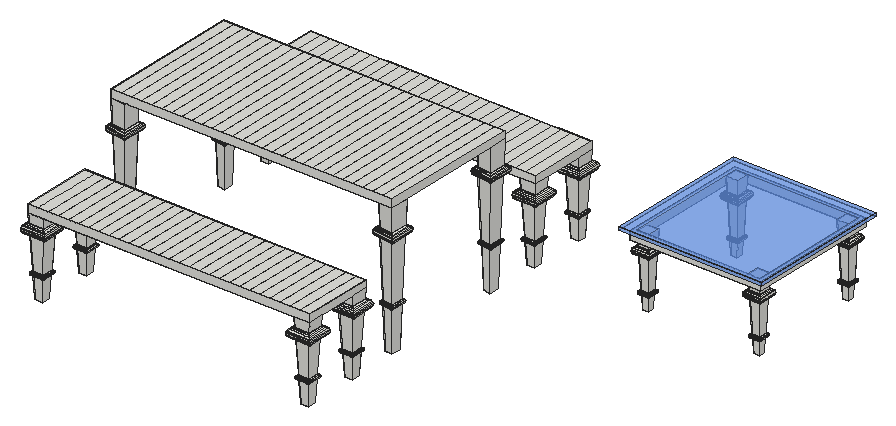
# SketchUp Ruby script. Lengths in millimetres.
U = 1.mm
M = Sketchup.active_model
def pt(a) = Geom::Point3d.new(a.map { |v| v * U })
def face(e, loops, mat)
  f = e.add_face(loops[0].map { |a| pt(a) })
  loops[1..].each { |l| e.add_face(l.map { |a| pt(a) }).erase! }
  f.material = f.back_material = mat if mat
  f
end
# faces: each face lists its corners as indices into pts; further lists are holes
def faces(e, pts, list, mat = nil) = list.each { |f| face(e, (f[0].is_a?(Array) ? f : [f]).map { |l| l.map { |i| pts[i] } }, mat) }
# xy, xz, yz: faces in a plane at the given z, y or x. An outline is a flat list of corners, or four numbers for a rectangle; further outlines are holes
def ring(l) = l.size == 4 ? [[l[0], l[1]], [l[2], l[1]], [l[2], l[3]], [l[0], l[3]]] : l.each_slice(2).to_a
def flat(e, list, mat, &to3) = list.each { |f| face(e, (f[0].is_a?(Array) ? f : [f]).map { |l| ring(l).map { |u, v| to3.(u, v) } }, mat) }
def xy(e, z, list, mat = nil) = flat(e, list, mat) { |x, y| [x, y, z] }
def xz(e, y, list, mat = nil) = flat(e, list, mat) { |x, z| [x, y, z] }
def yz(e, x, list, mat = nil) = flat(e, list, mat) { |y, z| [x, y, z] }
def lines(e, pts, list) = list.each { |a, b| e.add_line(pt(pts[a]), pt(pts[b])) }
# prism: a flat outline (further loops are holes) pulled along v
def prism(e, loops, v, mat = nil)
  f = face(e, loops, mat); d = Geom::Vector3d.new(v.map { |x| x * U })
  f.pushpull(f.normal.samedirection?(d) ? d.length : -d.length)
end
def box(e, o, s, mat = nil) = prism(e, [[o, [o[0] + s[0], o[1], o[2]], [o[0] + s[0], o[1] + s[1], o[2]], [o[0], o[1] + s[1], o[2]]]], [0, 0, s[2]], mat)
def at(x, y, z, deg = 0) = Geom::Transformation.translation(pt([x, y, z])) * Geom::Transformation.rotation(ORIGIN, Z_AXIS, deg.degrees)
def axes(o, x, y, z) = Geom::Transformation.new([*x, 0, *y, 0, *z, 0, *pt(o).to_a, 1])
def part(name) = M.definitions.add(name)
# library, detail: a bought-in or finely detailed component or shape, given as its bounding box
def library(name, o, s) = part(name).tap { |d| box(d.entities, o, s) }
def detail(e, o, s) = box(e.add_group.entities, o, s)
def put(e, d, t, mat = nil) = e.add_instance(d, t).tap { |i| i.material = mat if mat }
def group(e, t, mat = nil) = e.add_group.tap { |g| g.transformation = t; g.material = mat if mat }.entities
root = M.entities
M.materials.add("[Translucent Glass Blue]").color = [100, 149, 237]
M.materials["[Translucent Glass Blue]"].alpha = 0.5
c1 = part("Table leg \#1")
xy(c1.entities,0,[[95.2,52.8,45.9,59.8,45.9,113.1,95.7,113.1]])
xy(c1.entities,858,[[120,24.1,120.9,138.1,20.9,138.1,20.9,38.1]])
p = [[38.2,53.1,264.1],[45.9,59.8,0],[95.2,52.8,0],[102.8,44,264.1],[95.7,113.1,0],[103.5,120.8,264.1],
  [38.2,120.8,264.1],[45.9,113.1,0],[34.7,50,264.4],[37.9,52.8,264],[103.2,43.6,264],[106.4,39.8,264.4],
  [103.9,121.1,264],[107.1,124.4,264.4],[34.7,124.4,264.4],[37.9,121.1,264],[31.6,47.3,265.7],[109.4,36.4,265.7],
  [110.2,127.4,265.7],[31.6,127.4,265.7],[29,45.1,267.7],[111.9,33.4,267.7],[112.8,130,267.7],[29,130,267.7],
  [27.1,43.4,270.2],[113.9,31.1,270.2],[114.8,131.9,270.2],[27.1,131.9,270.2],[25.8,42.3,273.3],[115.1,29.7,273.3],
  [116,133.2,273.3],[25.8,133.2,273.3],[25.4,41.9,276.5],[115.6,29.2,276.5],[116.5,133.6,276.5],[25.4,133.6,276.5],
  [25.8,42.3,279.7],[115.1,29.7,279.7],[116,133.2,279.7],[25.8,133.2,279.7],[27.1,43.4,282.7],[113.9,31.1,282.7],
  [114.8,131.9,282.7],[27.1,131.9,282.7],[29,45.1,285.3],[111.9,33.4,285.3],[112.8,130,285.3],[29,130,285.3],
  [31.6,47.3,287.3],[109.4,36.4,287.3],[110.2,127.4,287.3],[31.6,127.4,287.3],[34.7,50,288.6],[106.4,39.8,288.6],
  [107.1,124.4,288.6],[34.7,124.4,288.6],[37.5,52.5,288.9],[103.5,43.1,288.9],[104.2,121.5,288.9],[37.5,121.5,288.9],
  [26.7,43.1,658.9],[114.2,30.7,658.9],[115.1,132.3,658.9],[26.7,132.3,658.9],[20,37.2,659.6],[120.9,23,659.6],
  [121.9,139,659.6],[20,139,659.6],[13.6,31.7,662],[127.2,15.7,662],[128.3,145.4,662],[13.6,145.4,662],
  [8.1,26.9,665.9],[132.6,9.4,665.9],[133.8,150.9,665.9],[8.1,150.9,665.9],[3.9,23.2,671.2],[136.9,4.4,671.2],
  [138.2,155.1,671.2],[3.9,155.1,671.2],[1.1,20.8,677.4],[139.6,1.2,677.4],[141,157.9,677.4],[1.1,157.9,677.4],
  [0,19.9,684.1],[140.7,0,684.1],[142.1,159,684.1],[0,159,684.1],[0.7,20.5,690.8],[140,0.8,690.8],
  [141.4,158.3,690.8],[0.7,158.3,690.8],[3.1,22.6,697.2],[137.6,3.6,697.2],[138.9,155.9,697.2],[3.1,155.9,697.2],
  [7.1,26,702.7],[133.7,8.1,702.7],[134.9,151.9,702.7],[7.1,151.9,702.7],[12.3,30.6,707],[128.5,14.2,707],
  [129.6,146.7,707],[12.3,146.7,707],[18.5,36,709.7],[122.3,21.3,709.7],[123.4,140.5,709.7],[18.5,140.5,709.7],
  [25.2,41.8,710.8],[115.7,29,710.8],[116.6,133.8,710.8],[25.2,133.8,710.8],[120,24.1,858],[20.9,38.1,858],
  [120.9,138.1,858],[20.9,138.1,858]]
faces(c1.entities,p,[[0,1,2,3],[4,5,3,2],[6,7,1,0],[5,4,7,6],[8,9,10,11],[11,10,12,13],[9,0,3,10],[10,3,5,12],
  [14,15,9,8],[15,6,0,9],[12,5,6,15],[13,12,15,14],[16,8,11,17],[17,11,13,18],[19,14,8,16],[18,13,14,19],
  [20,16,17,21],[21,17,18,22],[23,19,16,20],[22,18,19,23],[24,20,21,25],[25,21,22,26],[27,23,20,24],[26,22,23,27],
  [28,24,25,29],[29,25,26,30],[31,27,24,28],[30,26,27,31],[32,28,29,33],[33,29,30,34],[35,31,28,32],[34,30,31,35],
  [36,32,33,37],[37,33,34,38],[39,35,32,36],[38,34,35,39],[40,36,37,41],[41,37,38,42],[43,39,36,40],[42,38,39,43],
  [44,40,41,45],[45,41,42,46],[47,43,40,44],[46,42,43,47],[48,44,45,49],[49,45,46,50],[51,47,44,48],[50,46,47,51],
  [52,48,49,53],[53,49,50,54],[55,51,48,52],[54,50,51,55],[56,52,53,57],[57,53,54,58],[59,55,52,56],[58,54,55,59],
  [60,56,57,61],[58,62,61,57],[63,59,56,60],[62,58,59,63],[64,60,61,65],[65,61,62,66],[67,63,60,64],[66,62,63,67],
  [68,64,65,69],[69,65,66,70],[71,67,64,68],[70,66,67,71],[72,68,69,73],[73,69,70,74],[75,71,68,72],[74,70,71,75],
  [76,72,73,77],[77,73,74,78],[79,75,72,76],[78,74,75,79],[80,76,77,81],[81,77,78,82],[83,79,76,80],[82,78,79,83],
  [84,80,81,85],[85,81,82,86],[87,83,80,84],[86,82,83,87],[88,84,85,89],[89,85,86,90],[91,87,84,88],[90,86,87,91],
  [92,88,89,93],[93,89,90,94],[95,91,88,92],[94,90,91,95],[96,92,93,97],[97,93,94,98],[99,95,92,96],[98,94,95,99],
  [100,96,97,101],[101,97,98,102],[103,99,96,100],[102,98,99,103],[104,100,101,105],[105,101,102,106],[107,103,100,104],[106,102,103,107],
  [108,104,105,109],[109,105,106,110],[111,107,104,108],[110,106,107,111],[109,112,113,108],[110,114,112,109],[108,113,115,111],[111,115,114,110]])
c2 = part("Bench leg")
xy(c2.entities,0,[[52.8,52.8,102.8,102.8]])
xy(c2.entities,500,[[27.8,27.8,127.8,127.8]])
p = [[102.8,52.8,0],[109.7,45.9,138.3],[45.9,45.9,138.3],[52.8,52.8,0],[45.9,109.7,138.3],[52.8,102.8,0],
  [102.8,102.8,0],[109.7,109.7,138.3],[42,113.6,138.6],[45.2,110.3,138.2],[45.2,45.2,138.2],[42,42,138.6],
  [110.3,45.2,138.2],[113.6,42,138.6],[110.3,110.3,138.2],[113.6,113.6,138.6],[39,116.6,139.9],[39,39,139.9],
  [116.6,39,139.9],[116.6,116.6,139.9],[36.4,119.2,141.9],[36.4,36.4,141.9],[119.2,36.4,141.9],[119.2,119.2,141.9],
  [34.4,121.1,144.4],[34.4,34.4,144.4],[121.1,34.4,144.4],[121.1,121.1,144.4],[33.2,122.4,147.5],[33.2,33.2,147.5],
  [122.4,33.2,147.5],[122.4,122.4,147.5],[32.7,32.7,150.7],[122.8,32.7,150.7],[32.7,122.8,150.7],[122.8,122.8,150.7],
  [33.2,122.4,153.9],[33.2,33.2,153.9],[122.4,33.2,153.9],[122.4,122.4,153.9],[34.4,121.1,156.9],[34.4,34.4,156.9],
  [121.1,34.4,156.9],[121.1,121.1,156.9],[36.4,119.2,159.5],[36.4,36.4,159.5],[119.2,36.4,159.5],[119.2,119.2,159.5],
  [39,116.6,161.5],[39,39,161.5],[116.6,39,161.5],[116.6,116.6,161.5],[42,113.6,162.7],[42,42,162.7],
  [113.6,42,162.7],[113.6,113.6,162.7],[44.6,110.9,163.1],[44.6,44.6,163.1],[110.9,44.6,163.1],[110.9,110.9,163.1],
  [121.5,34,374.9],[34,34,374.9],[34,121.5,374.9],[121.5,121.5,374.9],[24,24,375.8],[32.4,32.4,374.6],
  [123.1,32.4,374.6],[131.5,24,375.8],[24,131.5,375.8],[32.4,123.1,374.6],[123.1,123.1,374.6],[131.5,131.5,375.8],
  [16.2,16.2,379],[139.4,16.2,379],[16.2,139.4,379],[139.4,139.4,379],[9.5,146.1,384.1],[9.5,9.5,384.1],
  [146.1,9.5,384.1],[146.1,146.1,384.1],[4.3,4.3,390.8],[151.2,4.3,390.8],[4.3,151.2,390.8],[151.2,151.2,390.8],
  [1.1,1.1,398.7],[154.5,1.1,398.7],[1.1,154.5,398.7],[154.5,154.5,398.7],[0,155.6,407],[0,0,407],
  [155.6,0,407],[155.6,155.6,407],[1.1,154.5,415.4],[1.1,1.1,415.4],[154.5,1.1,415.4],[154.5,154.5,415.4],
  [4.3,151.2,423.2],[4.3,4.3,423.2],[151.2,4.3,423.2],[151.2,151.2,423.2],[9.5,9.5,429.9],[146.1,9.5,429.9],
  [9.5,146.1,429.9],[146.1,146.1,429.9],[16.2,139.4,435.1],[16.2,16.2,435.1],[139.4,16.2,435.1],[139.4,139.4,435.1],
  [24,131.5,438.3],[24,24,438.3],[131.5,24,438.3],[131.5,131.5,438.3],[30.8,124.7,439.2],[30.8,30.8,439.2],
  [124.7,30.8,439.2],[124.7,124.7,439.2],[27.8,27.8,500],[27.8,127.8,500],[127.8,27.8,500],[127.8,127.8,500]]
faces(c2.entities,p,[[0,1,2,3],[4,5,3,2],[6,7,1,0],[7,6,5,4],[8,9,10,11],[11,10,12,13],[13,12,14,15],[9,4,2,10],
  [10,2,1,12],[12,1,7,14],[14,7,4,9],[15,14,9,8],[16,8,11,17],[17,11,13,18],[18,13,15,19],[19,15,8,16],
  [20,16,17,21],[21,17,18,22],[22,18,19,23],[23,19,16,20],[24,20,21,25],[25,21,22,26],[26,22,23,27],[27,23,20,24],
  [28,24,25,29],[29,25,26,30],[30,26,27,31],[31,27,24,28],[32,29,30,33],[34,28,29,32],[33,30,31,35],[35,31,28,34],
  [36,34,32,37],[37,32,33,38],[38,33,35,39],[39,35,34,36],[40,36,37,41],[41,37,38,42],[42,38,39,43],[43,39,36,40],
  [44,40,41,45],[45,41,42,46],[46,42,43,47],[47,43,40,44],[48,44,45,49],[49,45,46,50],[50,46,47,51],[51,47,44,48],
  [52,48,49,53],[53,49,50,54],[54,50,51,55],[55,51,48,52],[56,52,53,57],[57,53,54,58],[58,54,55,59],[59,55,52,56],
  [58,60,61,57],[62,56,57,61],[59,63,60,58],[56,62,63,59],[64,65,66,67],[68,69,65,64],[67,66,70,71],[69,62,61,65],
  [65,61,60,66],[66,60,63,70],[70,63,62,69],[71,70,69,68],[72,64,67,73],[74,68,64,72],[73,67,71,75],[75,71,68,74],
  [76,74,72,77],[77,72,73,78],[78,73,75,79],[79,75,74,76],[80,77,78,81],[82,76,77,80],[81,78,79,83],[83,79,76,82],
  [84,80,81,85],[86,82,80,84],[85,81,83,87],[87,83,82,86],[88,86,84,89],[89,84,85,90],[90,85,87,91],[91,87,86,88],
  [92,88,89,93],[93,89,90,94],[94,90,91,95],[95,91,88,92],[96,92,93,97],[97,93,94,98],[98,94,95,99],[99,95,92,96],
  [100,97,98,101],[102,96,97,100],[101,98,99,103],[103,99,96,102],[104,102,100,105],[105,100,101,106],[106,101,103,107],[107,103,102,104],
  [108,104,105,109],[109,105,106,110],[110,106,107,111],[111,107,104,108],[112,108,109,113],[113,109,110,114],[114,110,111,115],[115,111,108,112],
  [113,116,117,112],[114,118,116,113],[115,119,118,114],[112,117,119,115]])
c3 = part("Square tabletop frame")
prism(c3.entities,[[[0,838.2,0],[838.2,838.2,0],[838.2,0,0],[0,0,0]],[[812.8,25.4,0],[812.8,812.8,0],[25.4,812.8,0],[25.4,25.4,0]]],[0,0,50.8])
c4 = part("Table leg")
xy(c4.entities,0,[[39.7,39.7,77.8,77.8]])
xy(c4.entities,88.3,[[35.5,35.5,35.5,82,36,81.4,36,36],[35.5,35.5,36,36,81.4,36,82,35.5],[82,35.5,81.4,36,81.4,81.4,82,82],[36,81.4,35.5,82,82,82,81.4,81.4]])
xy(c4.entities,457.2,[[20.6,20.6,96.8,96.8]])
p = [[39.7,39.7,0],[36,36,88.3],[36,81.4,88.3],[39.7,77.8,0],[77.8,39.7,0],[81.4,36,88.3],
  [77.8,77.8,0],[81.4,81.4,88.3],[32.2,32.2,88.7],[35.5,35.5,88.3],[82,35.5,88.3],[85.3,32.2,88.7],
  [32.2,85.3,88.7],[35.5,82,88.3],[82,82,88.3],[85.3,85.3,88.7],[29.1,29.1,90],[88.3,29.1,90],
  [29.1,88.3,90],[88.3,88.3,90],[26.5,26.5,92],[91,26.5,92],[26.5,91,92],[91,91,92],
  [24.5,93,94.6],[24.5,24.5,94.6],[93,24.5,94.6],[93,93,94.6],[23.2,94.2,97.7],[23.2,23.2,97.7],
  [94.2,23.2,97.7],[94.2,94.2,97.7],[22.8,22.8,101],[94.7,22.8,101],[22.8,94.7,101],[94.7,94.7,101],
  [23.2,23.2,104.3],[94.2,23.2,104.3],[23.2,94.2,104.3],[94.2,94.2,104.3],[24.5,24.5,107.3],[93,24.5,107.3],
  [24.5,93,107.3],[93,93,107.3],[26.5,26.5,109.9],[91,26.5,109.9],[26.5,91,109.9],[91,91,109.9],
  [29.1,29.1,112],[88.3,29.1,112],[29.1,88.3,112],[88.3,88.3,112],[32.2,32.2,113.2],[85.3,32.2,113.2],
  [32.2,85.3,113.2],[85.3,85.3,113.2],[34.9,34.9,113.6],[82.5,34.9,113.6],[34.9,82.5,113.6],[82.5,82.5,113.6],
  [26.5,26.5,317.1],[26.5,91,317.1],[91,26.5,317.1],[91,91,317.1],[18.8,98.6,317.9],[25.4,92,317],
  [25.4,25.4,317],[18.8,18.8,317.9],[92,25.4,317],[98.6,18.8,317.9],[92,92,317],[98.6,98.6,317.9],
  [12.7,104.7,320.4],[12.7,12.7,320.4],[104.7,12.7,320.4],[104.7,104.7,320.4],[7.4,110,324.4],[7.4,7.4,324.4],
  [110,7.4,324.4],[110,110,324.4],[3.4,114,329.7],[3.4,3.4,329.7],[114,3.4,329.7],[114,114,329.7],
  [0.9,116.6,335.8],[0.9,0.9,335.8],[116.6,0.9,335.8],[116.6,116.6,335.8],[0,117.4,342.4],[0,0,342.4],
  [117.4,0,342.4],[117.4,117.4,342.4],[0.9,116.6,348.9],[0.9,0.9,348.9],[116.6,0.9,348.9],[116.6,116.6,348.9],
  [3.4,114,355.1],[3.4,3.4,355.1],[114,3.4,355.1],[114,114,355.1],[7.4,7.4,360.3],[110,7.4,360.3],
  [7.4,110,360.3],[110,110,360.3],[12.7,12.7,364.3],[104.7,12.7,364.3],[12.7,104.7,364.3],[104.7,104.7,364.3],
  [18.8,98.6,366.9],[18.8,18.8,366.9],[98.6,18.8,366.9],[98.6,98.6,366.9],[24.3,93.1,367.6],[24.3,24.3,367.6],
  [93.1,24.3,367.6],[93.1,93.1,367.6],[20.6,20.6,457.2],[20.6,96.8,457.2],[96.8,20.6,457.2],[96.8,96.8,457.2]]
faces(c4.entities,p,[[0,1,2,3],[1,0,4,5],[6,7,5,4],[7,6,3,2],[8,9,10,11],[12,13,9,8],[11,10,14,15],[15,14,13,12],
  [16,8,11,17],[18,12,8,16],[17,11,15,19],[19,15,12,18],[20,16,17,21],[22,18,16,20],[21,17,19,23],[23,19,18,22],
  [24,22,20,25],[25,20,21,26],[26,21,23,27],[27,23,22,24],[28,24,25,29],[29,25,26,30],[30,26,27,31],[31,27,24,28],
  [32,29,30,33],[34,28,29,32],[33,30,31,35],[35,31,28,34],[36,32,33,37],[38,34,32,36],[37,33,35,39],[39,35,34,38],
  [40,36,37,41],[42,38,36,40],[41,37,39,43],[43,39,38,42],[44,40,41,45],[46,42,40,44],[45,41,43,47],[47,43,42,46],
  [48,44,45,49],[50,46,44,48],[49,45,47,51],[51,47,46,50],[52,48,49,53],[54,50,48,52],[53,49,51,55],[55,51,50,54],
  [56,52,53,57],[58,54,52,56],[57,53,55,59],[59,55,54,58],[56,60,61,58],[57,62,60,56],[59,63,62,57],[63,59,58,61],
  [64,65,66,67],[67,66,68,69],[69,68,70,71],[65,61,60,66],[66,60,62,68],[68,62,63,70],[70,63,61,65],[71,70,65,64],
  [72,64,67,73],[73,67,69,74],[74,69,71,75],[75,71,64,72],[76,72,73,77],[77,73,74,78],[78,74,75,79],[79,75,72,76],
  [80,76,77,81],[81,77,78,82],[82,78,79,83],[83,79,76,80],[84,80,81,85],[85,81,82,86],[86,82,83,87],[87,83,80,84],
  [88,84,85,89],[89,85,86,90],[90,86,87,91],[91,87,84,88],[92,88,89,93],[93,89,90,94],[94,90,91,95],[95,91,88,92],
  [96,92,93,97],[97,93,94,98],[98,94,95,99],[99,95,92,96],[100,97,98,101],[102,96,97,100],[101,98,99,103],[103,99,96,102],
  [104,100,101,105],[106,102,100,104],[105,101,103,107],[107,103,102,106],[108,106,104,109],[109,104,105,110],[110,105,107,111],[111,107,106,108],
  [112,108,109,113],[113,109,110,114],[114,110,111,115],[115,111,108,112],[113,116,117,112],[114,118,116,113],[115,119,118,114],[112,117,119,115]])
xy(root,1894.5,[[2888.6,1180.6,3803,2095]],"[Translucent Glass Blue]")
xy(root,1919.9,[[2888.6,1180.6,3803,2095]],"[Translucent Glass Blue]")
xz(root,1180.6,[[2888.6,1894.5,3803,1919.9]],"[Translucent Glass Blue]")
xz(root,2095,[[2888.6,1894.5,3803,1919.9]],"[Translucent Glass Blue]")
yz(root,2888.6,[[1180.6,1894.5,2095,1919.9]],"[Translucent Glass Blue]")
yz(root,3803,[[1180.6,1894.5,2095,1919.9]],"[Translucent Glass Blue]")
p = [[27.8,1590.9,1919.9],[27.8,690.9,1919.9],[92.1,1590.9,1919.9],[92.1,690.9,1919.9],[156.4,1590.9,1919.9],[156.4,690.9,1919.9],
  [220.6,1590.9,1919.9],[220.6,690.9,1919.9],[284.9,1590.9,1919.9],[284.9,690.9,1919.9],[349.2,1590.9,1919.9],[349.2,690.9,1919.9],
  [413.5,1590.9,1919.9],[413.5,690.9,1919.9],[477.8,1590.9,1919.9],[477.8,690.9,1919.9],[542.1,1590.9,1919.9],[542.1,690.9,1919.9],
  [606.4,1590.9,1919.9],[606.4,690.9,1919.9],[670.6,1590.9,1919.9],[670.6,690.9,1919.9],[734.9,1590.9,1919.9],[734.9,690.9,1919.9],
  [799.2,1590.9,1919.9],[799.2,690.9,1919.9],[863.5,1590.9,1919.9],[863.5,690.9,1919.9],[927.8,1590.9,1919.9],[927.8,690.9,1919.9],
  [992.1,1590.9,1919.9],[992.1,690.9,1919.9],[1056.4,1590.9,1919.9],[1056.4,690.9,1919.9],[1120.6,1590.9,1919.9],[1120.6,690.9,1919.9],
  [1184.9,1590.9,1919.9],[1184.9,690.9,1919.9],[1249.2,1590.9,1919.9],[1249.2,690.9,1919.9],[1313.5,1590.9,1919.9],[1313.5,690.9,1919.9],
  [1377.8,1590.9,1919.9],[1377.8,690.9,1919.9],[1442.1,1590.9,1919.9],[1442.1,690.9,1919.9],[1506.4,1590.9,1919.9],[1506.4,690.9,1919.9],
  [1570.6,1590.9,1919.9],[1570.6,690.9,1919.9],[1634.9,1590.9,1919.9],[1634.9,690.9,1919.9],[1699.2,1590.9,1919.9],[1699.2,690.9,1919.9],
  [1763.5,1590.9,1919.9],[1763.5,690.9,1919.9],[1402.4,6474.7,-581.5],[1402.4,6474.5,-587.5]]
lines(root,p,[[0,1],[2,3],[4,5],[6,7],[8,9],[10,11],[12,13],[14,15],[16,17],[18,19],[20,21],[22,23],
  [24,25],[26,27],[28,29],[30,31],[32,33],[34,35],[36,37],[38,39],[40,41],[42,43],[44,45],[46,47],
  [48,49],[50,51],[52,53],[54,55],[56,57]])
put(root,c1,at(1707.8,666.8,1011.9))
put(root,c1,at(1707.8,1452.9,1011.9))
put(root,c1,at(6.8,1452.9,1011.9))
put(root,c1,at(6.8,652.9,1011.9))
put(root,c2,at(0,0,1003.2))
put(root,c2,at(1700,0,1003.2))
put(root,c2,at(1700,350,1003.2))
put(root,c2,at(0,350,1003.2))
put(root,c2,at(0,1809,1003.2))
put(root,c2,at(1700,1809,1003.2))
put(root,c2,at(1700,2159,1003.2))
put(root,c2,at(0,2159,1003.2))
put(root,c3,at(2926.7,1218.7,1843.7))
put(root,c4,at(2931.5,1223.5,1437.3))
put(root,c4,at(3642.7,1934.7,1437.3))
put(root,c4,at(3642.7,1223.5,1437.3))
put(root,c4,at(2931.5,1934.7,1437.3))
g1 = group(root,at(27.8,690.9,1869.9))
box(g1,[0,0,0],[1800,900,50])
g2 = group(root,at(27.8,27.8,1503.2))
xy(g2,0,[[0,0,1800,450]])
xy(g2,50,[[0,0,64,0,64,0.4,0,1],[64,0,1800,0,1800,450,68,450,64,0.4],[64,0.4,68,450,0,450,0,1]])
xz(g2,0,[[0,0,1800,50]])
xz(g2,450,[[0,0,1800,50]])
yz(g2,0,[[0,0,450,50]])
yz(g2,1800,[[0,0,450,50]])
p = [[128.3,0.4,50],[132.3,450,50],[192.6,0.4,50],[196.5,450,50],[256.9,0.4,50],[260.8,450,50],
  [321.2,0.4,50],[325.1,450,50],[385.5,0.4,50],[389.4,450,50],[449.8,0.4,50],[453.7,450,50],
  [514.1,0.4,50],[518,450,50],[578.4,0.4,50],[582.3,450,50],[642.7,0.4,50],[646.6,450,50],
  [707,0.4,50],[710.9,450,50],[771.3,0.4,50],[775.2,450,50],[835.6,0.4,50],[839.5,450,50],
  [899.9,0.4,50],[903.8,450,50],[964.1,0.4,50],[968.1,450,50],[1028.4,0.4,50],[1032.4,450,50],
  [1092.7,0.4,50],[1096.7,450,50],[1157,0.4,50],[1161,450,50],[1221.3,0.4,50],[1225.3,450,50],
  [1285.6,0.4,50],[1289.6,450,50],[1349.9,0.4,50],[1353.9,450,50],[1414.2,0.4,50],[1418.2,450,50],
  [1478.5,0.4,50],[1482.5,450,50],[1542.8,0.4,50],[1546.8,450,50],[1607.1,0.4,50],[1611.1,450,50],
  [1671.4,0.4,50],[1675.4,450,50],[1735.7,0.4,50],[1739.7,450,50],[1800,0.4,50],[1804,450,50]]
lines(g2,p,[[0,1],[2,3],[4,5],[6,7],[8,9],[10,11],[12,13],[14,15],[16,17],[18,19],[20,21],[22,23],
  [24,25],[26,27],[28,29],[30,31],[32,33],[34,35],[36,37],[38,39],[40,41],[42,43],[44,45],[46,47],
  [48,49],[50,51],[52,53]])
g3 = group(root,at(27.8,1836.8,1503.2))
prism(g3,[[[0,0,0],[1800,0,0],[1800,0,50],[1736,0,50],[1671.7,0,50],[1607.4,0,50],[1543.1,0,50],[1478.8,0,50],[1414.5,0,50],[1350.2,0,50],[1285.9,0,50],[1221.6,0,50],[1157.3,0,50],[1093,0,50],[1028.7,0,50],[964.4,0,50],[900.1,0,50],[835.9,0,50],[771.6,0,50],[707.3,0,50],[643,0,50],[578.7,0,50],[514.4,0,50],[450.1,0,50],[385.8,0,50],[321.5,0,50],[257.2,0,50],[192.9,0,50],[128.6,0,50],[64.3,0,50],[0,0,50]]],[0,450,0])
